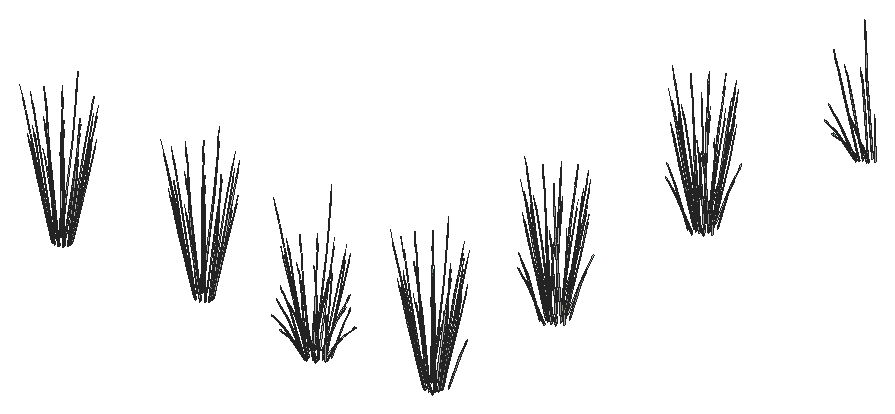
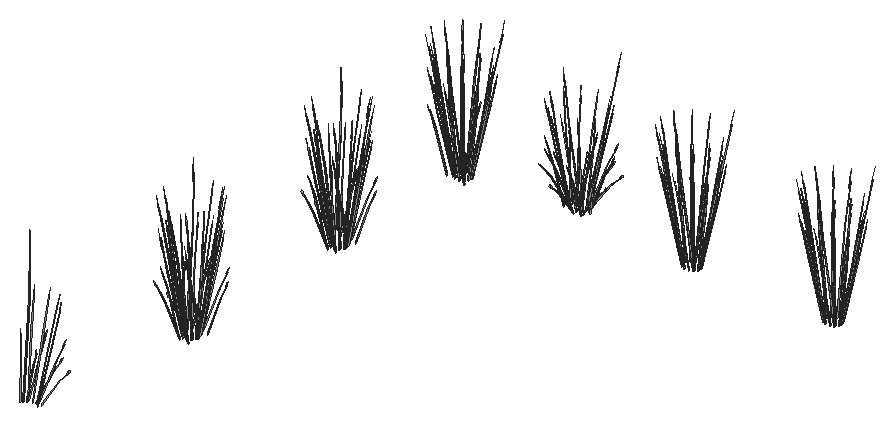
# SketchUp Ruby script. Lengths in inches.
U = 1.inch
M = Sketchup.active_model
def pt(a) = Geom::Point3d.new(a.map { |v| v * U })
def face(e, loops, mat)
  f = e.add_face(loops[0].map { |a| pt(a) })
  loops[1..].each { |l| e.add_face(l.map { |a| pt(a) }).erase! }
  f.material = f.back_material = mat if mat
  f
end
# faces: each face lists its corners as indices into pts; further lists are holes
def faces(e, pts, list, mat = nil) = list.each { |f| face(e, (f[0].is_a?(Array) ? f : [f]).map { |l| l.map { |i| pts[i] } }, mat) }
# xy, xz, yz: faces in a plane at the given z, y or x. An outline is a flat list of corners, or four numbers for a rectangle; further outlines are holes
def ring(l) = l.size == 4 ? [[l[0], l[1]], [l[2], l[1]], [l[2], l[3]], [l[0], l[3]]] : l.each_slice(2).to_a
def flat(e, list, mat, &to3) = list.each { |f| face(e, (f[0].is_a?(Array) ? f : [f]).map { |l| ring(l).map { |u, v| to3.(u, v) } }, mat) }
def xy(e, z, list, mat = nil) = flat(e, list, mat) { |x, y| [x, y, z] }
def xz(e, y, list, mat = nil) = flat(e, list, mat) { |x, z| [x, y, z] }
def yz(e, x, list, mat = nil) = flat(e, list, mat) { |y, z| [x, y, z] }
def lines(e, pts, list) = list.each { |a, b| e.add_line(pt(pts[a]), pt(pts[b])) }
# prism: a flat outline (further loops are holes) pulled along v
def prism(e, loops, v, mat = nil)
  f = face(e, loops, mat); d = Geom::Vector3d.new(v.map { |x| x * U })
  f.pushpull(f.normal.samedirection?(d) ? d.length : -d.length)
end
def box(e, o, s, mat = nil) = prism(e, [[o, [o[0] + s[0], o[1], o[2]], [o[0] + s[0], o[1] + s[1], o[2]], [o[0], o[1] + s[1], o[2]]]], [0, 0, s[2]], mat)
def at(x, y, z, deg = 0) = Geom::Transformation.translation(pt([x, y, z])) * Geom::Transformation.rotation(ORIGIN, Z_AXIS, deg.degrees)
def axes(o, x, y, z) = Geom::Transformation.new([*x, 0, *y, 0, *z, 0, *pt(o).to_a, 1])
def part(name) = M.definitions.add(name)
# library, detail: a bought-in or finely detailed component or shape, given as its bounding box
def library(name, o, s) = part(name).tap { |d| box(d.entities, o, s) }
def detail(e, o, s) = box(e.add_group.entities, o, s)
def put(e, d, t, mat = nil) = e.add_instance(d, t).tap { |i| i.material = mat if mat }
def group(e, t, mat = nil) = e.add_group.tap { |g| g.transformation = t; g.material = mat if mat }.entities
root = M.entities
M.materials.add("LightPink_Translucent").color = [175, 214, 192]
M.materials["LightPink_Translucent"].alpha = 0.75
c1 = part("blade")
p = [[2.15,0.21,22],[0,0.17,0],[0.09,0.45,0],[2.18,0.31,22],[2.29,0.31,22],[0.38,0.45,0],
  [2.48,0.24,33],[2.49,0.24,33],[2.48,0.22,33]]
faces(c1.entities,p,[[0,1,2,3],[4,5,2,3],[6,3,4,7],[8,0,3,6]])
c2 = part("seeds")
p = [[0.3,-0.1,1.38],[-0.01,-0.03,1.59],[-0.01,-0.03,0.03],[0.14,-0.07,-0.07],[0.29,-0.03,3],[0.15,0.01,3.11]]
faces(c2.entities,p,[[0,1,2,3],[1,0,4,5]],"LightPink_Translucent")
c3 = part("blade with seeds")
put(c3.entities,c1,at(0,0,0))
put(c3.entities,c2,axes([2.4,0.25,30.99],[1.5799,-0.05474,1.17369],[-0.12525,1.92788,0.29478],[-0.07173,-0.02425,1.56792]))
put(root,c3,axes([463.08,228.78,141.56],[-0.0731,-0.06244,1.59199],[-0.48785,0.03959,-0.25177],[-0.07786,-0.14934,0.12768]))
put(root,c3,axes([465.27,229.54,141.56],[-0.00461,-0.08863,1.59199],[-0.38966,-0.25616,-0.25177],[0.06024,-0.15528,0.12768]))
put(root,c3,axes([465.17,229.22,141.55],[-0.04854,0.03402,1.61419],[-0.47555,-0.11476,-0.15253],[-0.01722,-0.14844,0.28566]))
put(root,c3,axes([462.58,228.57,141.55],[-0.00892,0.05338,1.61419],[-0.43976,0.19372,-0.15253],[-0.12941,-0.09903,0.28566]))
put(root,c3,axes([463.81,229.57,141.57],[0.35217,-0.15135,0.05852],[0.17238,0.27599,0.46065],[-0.03401,-0.12166,0.70242]))
put(root,c3,axes([462.6,229.61,141.57],[0.21722,-0.2829,0.05852],[0.30933,0.1647,0.46065],[-0.10001,-0.0907,0.70242]))
put(root,c3,axes([462.7,229.59,142.21],[-0.31898,0.42693,-0.12394],[-0.46194,-0.24596,-0.6879],[-0.16057,-0.12062,1.04526]))
put(root,c3,axes([464.88,230.06,141.57],[0.39276,0.02075,0.05852],[-0.01077,0.31333,0.46065],[0.0411,-0.12002,0.70242]))
put(root,c3,axes([461.48,229.46,141.56],[-0.10283,-0.00314,1.59199],[-0.32739,0.31434,-0.25177],[-0.17468,-0.06423,0.12768]))
put(root,c3,axes([466.45,230.92,141.55],[-0.06243,-0.00338,1.61419],[-0.25923,-0.3624,-0.15253],[0.1041,-0.11916,0.28566]))
put(root,c3,axes([461.58,230.17,141.57],[0.02407,-0.33864,0.05852],[0.3634,0.00928,0.46065],[-0.13921,-0.03543,0.70242]))
put(root,c3,axes([465.52,230.9375,141.57],[0.32811,0.18729,0.05852],[-0.19103,0.26671,0.46065],[0.10519,-0.08623,0.70242]))
put(root,c3,axes([466.6875,231.35,141.56],[0.06632,-0.06783,1.59199],[-0.08489,-0.4161,-0.25177],[0.16641,-0.07889,0.12768]))
put(root,c3,axes([461.08,229.73,141.55],[0.03543,0.04444,1.61419],[-0.17081,0.3995,-0.15253],[-0.17299,0.00289,0.28566]))
put(root,c3,axes([461.02,231.09,141.57],[-0.17554,-0.30365,0.05852],[0.3201,-0.14862,0.46065],[-0.1411,0.02932,0.70242]))
put(root,c3,axes([492.89,234.04,141.46],[-0.04854,0.03402,1.61419],[-0.47555,-0.11476,-0.15253],[-0.01722,-0.14844,0.28566]))
put(root,c3,axes([465.57,231.98,141.57],[0.17554,0.30365,0.05852],[-0.3201,0.14862,0.46065],[0.1411,-0.02932,0.70242]))
put(root,c3,axes([391.2,234.42,141.48],[0.47094,0.11642,0.43682],[-0.16104,0.38276,0.36018],[-0.0283,-0.15052,0.9039]))
put(root,c3,axes([429.4,234.42,141.48],[0.47094,0.11642,0.43682],[-0.16104,0.38276,0.36018],[-0.0283,-0.15052,0.9039]))
put(root,c3,axes([491.41,234.42,141.48],[0.47094,0.11642,0.43682],[-0.16104,0.38276,0.36018],[-0.0283,-0.15052,0.9039]))
put(root,c3,axes([391.33,234.39,141.47],[0.35217,-0.15135,0.05852],[0.17238,0.27599,0.46065],[-0.03401,-0.12166,0.70242]))
put(root,c3,axes([429.52,234.39,141.47],[0.35217,-0.15135,0.05852],[0.17238,0.27599,0.46065],[-0.03401,-0.12166,0.70242]))
put(root,c3,axes([491.53,234.39,141.47],[0.35217,-0.15135,0.05852],[0.17238,0.27599,0.46065],[-0.03401,-0.12166,0.70242]))
put(root,c3,axes([390.12,234.43,141.47],[0.21722,-0.2829,0.05852],[0.30933,0.1647,0.46065],[-0.10001,-0.0907,0.70242]))
put(root,c3,axes([428.32,234.43,141.47],[0.21722,-0.2829,0.05852],[0.30933,0.1647,0.46065],[-0.10001,-0.0907,0.70242]))
put(root,c3,axes([490.33,234.43,141.47],[0.21722,-0.2829,0.05852],[0.30933,0.1647,0.46065],[-0.10001,-0.0907,0.70242]))
put(root,c3,axes([466.34,233.18,141.55],[-0.04322,-0.03899,1.61419],[0.09454,-0.41791,-0.15253],[0.17023,-0.0267,0.28566]))
put(root,c3,axes([460.71,231.49,141.56],[-0.07805,0.05782,1.59199],[0.00664,0.42244,-0.25177],[-0.1789,0.05494,0.12768]))
put(root,c3,axes([392.27,234.84,141.48],[0.34034,0.30385,0.43682],[-0.36143,0.26205,0.36018],[0.06278,-0.14256,0.9039]))
put(root,c3,axes([430.47,234.84,141.48],[0.34034,0.30385,0.43682],[-0.36143,0.26205,0.36018],[0.06278,-0.14256,0.9039]))
put(root,c3,axes([492.48,234.84,141.48],[0.34034,0.30385,0.43682],[-0.36143,0.26205,0.36018],[0.06278,-0.14256,0.9039]))
put(root,c3,axes([390.22,234.4,142.11],[-0.31898,0.42693,-0.12394],[-0.46194,-0.24596,-0.6879],[-0.16057,-0.12062,1.04526]))
put(root,c3,axes([428.41,234.4,142.11],[-0.31898,0.42693,-0.12394],[-0.46194,-0.24596,-0.6879],[-0.16057,-0.12062,1.04526]))
put(root,c3,axes([490.42,234.4,142.11],[-0.31898,0.42693,-0.12394],[-0.46194,-0.24596,-0.6879],[-0.16057,-0.12062,1.04526]))
put(root,c3,axes([392.4,234.875,141.47],[0.39276,0.02075,0.05852],[-0.01077,0.31333,0.46065],[0.0411,-0.12002,0.70242]))
put(root,c3,axes([430.59,234.875,141.47],[0.39276,0.02075,0.05852],[-0.01077,0.31333,0.46065],[0.0411,-0.12002,0.70242]))
put(root,c3,axes([492.6,234.875,141.47],[0.39276,0.02075,0.05852],[-0.01077,0.31333,0.46065],[0.0411,-0.12002,0.70242]))
put(root,c3,axes([465.26,232.55,141.56],[0.10253,-0.00753,1.59199],[0.28122,-0.34598,-0.25177],[0.18237,0.04567,0.12768]))
put(root,c3,axes([461.07,232.13,141.57],[-0.32811,-0.18729,0.05852],[0.19103,-0.26671,0.46065],[-0.10519,0.08623,0.70242]))
put(root,c3,axes([389.1,234.99,141.47],[0.02407,-0.33864,0.05852],[0.3634,0.00928,0.46065],[-0.13921,-0.03543,0.70242]))
put(root,c3,axes([427.3,234.99,141.47],[0.02407,-0.33864,0.05852],[0.3634,0.00928,0.46065],[-0.13921,-0.03543,0.70242]))
put(root,c3,axes([489.31,234.99,141.47],[0.02407,-0.33864,0.05852],[0.3634,0.00928,0.46065],[-0.13921,-0.03543,0.70242]))
put(root,c3,axes([459.85,231.91,141.55],[0.061,0.01194,1.61419],[0.18869,0.39348,-0.15253],[-0.12486,0.10328,0.28566]))
put(root,c3,axes([465.01,232.9,141.57],[-0.02407,0.33864,0.05852],[-0.3634,-0.00928,0.46065],[0.13921,0.03543,0.70242]))
put(root,c3,axes([393.04,235.75,141.47],[0.32811,0.18729,0.05852],[-0.19103,0.26671,0.46065],[0.10519,-0.08623,0.70242]))
put(root,c3,axes([431.24,235.75,141.47],[0.32811,0.18729,0.05852],[-0.19103,0.26671,0.46065],[0.10519,-0.08623,0.70242]))
put(root,c3,axes([493.25,235.75,141.47],[0.32811,0.18729,0.05852],[-0.19103,0.26671,0.46065],[0.10519,-0.08623,0.70242]))
put(root,c3,axes([392.95,235.67,141.48],[0.11853,0.40986,0.43682],[-0.46497,0.07113,0.36018],[0.13704,-0.09639,0.9039]))
put(root,c3,axes([431.15,235.67,141.48],[0.11853,0.40986,0.43682],[-0.46497,0.07113,0.36018],[0.13704,-0.09639,0.9039]))
put(root,c3,axes([493.16,235.67,141.48],[0.11853,0.40986,0.43682],[-0.46497,0.07113,0.36018],[0.13704,-0.09639,0.9039]))
put(root,c3,axes([463.51,233.63,141.55],[0.00141,-0.05392,1.61419],[0.40958,-0.23787,-0.15253],[0.14227,0.0849,0.28566]))
put(root,c3,axes([461.72,233.01,141.57],[-0.39276,-0.02075,0.05852],[0.01077,-0.31333,0.46065],[-0.0411,0.12002,0.70242]))
put(root,c3,axes([463.99,233.45,141.57],[-0.21722,0.2829,0.05852],[-0.30933,-0.1647,0.46065],[0.10001,0.0907,0.70242]))
put(root,c3,axes([462.79,233.5,141.57],[-0.35217,0.15135,0.05852],[-0.17238,-0.27599,0.46065],[0.03401,0.12166,0.70242]))
put(root,c3,axes([460.73,233.0625,141.56],[-0.01188,0.08813,1.59199],[0.33715,0.30658,-0.25177],[-0.08826,0.14498,0.12768]))
put(root,c3,axes([461.8,232.87,142.18],[0.52527,0.02206,-0.12283],[-0.01436,0.41777,-0.68176],[-0.03649,0.1609,1.03593]))
put(root,c3,axes([388.57,236.02,141.48],[0.13503,-0.40605,0.43682],[0.44393,0.13885,0.36018],[-0.17458,0.0244,0.9039]))
put(root,c3,axes([426.77,236.02,141.48],[0.13503,-0.40605,0.43682],[0.44393,0.13885,0.36018],[-0.17458,0.0244,0.9039]))
put(root,c3,axes([488.78,236.02,141.48],[0.13503,-0.40605,0.43682],[0.44393,0.13885,0.36018],[-0.17458,0.0244,0.9039]))
put(root,c3,axes([388.54,235.91,141.47],[-0.17554,-0.30365,0.05852],[0.3201,-0.14862,0.46065],[-0.1411,0.02932,0.70242]))
put(root,c3,axes([426.73,235.91,141.47],[-0.17554,-0.30365,0.05852],[0.3201,-0.14862,0.46065],[-0.1411,0.02932,0.70242]))
put(root,c3,axes([488.75,235.91,141.47],[-0.17554,-0.30365,0.05852],[0.3201,-0.14862,0.46065],[-0.1411,0.02932,0.70242]))
put(root,c3,axes([460.6875,233.97,141.55],[0.05422,-0.02689,1.61419],[0.44816,0.17884,-0.15253],[-0.01053,0.14891,0.28566]))
put(root,c3,axes([393.09,236.79,141.47],[0.17554,0.30365,0.05852],[-0.3201,0.14862,0.46065],[0.1411,-0.02932,0.70242]))
put(root,c3,axes([431.29,236.79,141.47],[0.17554,0.30365,0.05852],[-0.3201,0.14862,0.46065],[0.1411,-0.02932,0.70242]))
put(root,c3,axes([493.3,236.79,141.47],[0.17554,0.30365,0.05852],[-0.3201,0.14862,0.46065],[0.1411,-0.02932,0.70242]))
put(root,c3,axes([393.06,236.6875,141.48],[-0.13503,0.40605,0.43682],[-0.44393,-0.13885,0.36018],[0.17458,-0.0244,0.9039]))
put(root,c3,axes([431.25,236.6875,141.48],[-0.13503,0.40605,0.43682],[-0.44393,-0.13885,0.36018],[0.17458,-0.0244,0.9039]))
put(root,c3,axes([493.26,236.6875,141.48],[-0.13503,0.40605,0.43682],[-0.44393,-0.13885,0.36018],[0.17458,-0.0244,0.9039]))
put(root,c3,axes([462.67,234.15,141.56],[0.06058,0.07171,1.59199],[0.48891,0.02817,-0.25177],[0.04916,0.15815,0.12768]))
put(root,c3,axes([494.0625,238,141.46],[-0.04322,-0.03899,1.61419],[0.09454,-0.41791,-0.15253],[0.17023,-0.0267,0.28566]))
put(root,c3,axes([388.68,237.03,141.48],[-0.11853,-0.40986,0.43682],[0.46497,-0.07113,0.36018],[-0.13704,0.09639,0.9039]))
put(root,c3,axes([426.875,237.03,141.48],[-0.11853,-0.40986,0.43682],[0.46497,-0.07113,0.36018],[-0.13704,0.09639,0.9039]))
put(root,c3,axes([488.89,237.03,141.48],[-0.11853,-0.40986,0.43682],[0.46497,-0.07113,0.36018],[-0.13704,0.09639,0.9039]))
put(root,c3,axes([388.59,236.95,141.47],[-0.32811,-0.18729,0.05852],[0.19103,-0.26671,0.46065],[-0.10519,0.08623,0.70242]))
put(root,c3,axes([426.78,236.95,141.47],[-0.32811,-0.18729,0.05852],[0.19103,-0.26671,0.46065],[-0.10519,0.08623,0.70242]))
put(root,c3,axes([488.79,236.95,141.47],[-0.32811,-0.18729,0.05852],[0.19103,-0.26671,0.46065],[-0.10519,0.08623,0.70242]))
put(root,c3,axes([392.53,237.72,141.47],[-0.02407,0.33864,0.05852],[-0.3634,-0.00928,0.46065],[0.13921,0.03543,0.70242]))
put(root,c3,axes([430.73,237.72,141.47],[-0.02407,0.33864,0.05852],[-0.3634,-0.00928,0.46065],[0.13921,0.03543,0.70242]))
put(root,c3,axes([492.74,237.72,141.47],[-0.02407,0.33864,0.05852],[-0.3634,-0.00928,0.46065],[0.13921,0.03543,0.70242]))
put(root,c3,axes([392.5625,237.61,141.48],[-0.35241,0.29344,0.43682],[-0.30393,-0.31162,0.36018],[0.16534,0.05413,0.9039]))
put(root,c3,axes([430.76,237.61,141.48],[-0.35241,0.29344,0.43682],[-0.30393,-0.31162,0.36018],[0.16534,0.05413,0.9039]))
put(root,c3,axes([492.77,237.61,141.48],[-0.35241,0.29344,0.43682],[-0.30393,-0.31162,0.36018],[0.16534,0.05413,0.9039]))
put(root,c3,axes([389.23,237.83,141.47],[-0.39276,-0.02075,0.05852],[0.01077,-0.31333,0.46065],[-0.0411,0.12002,0.70242]))
put(root,c3,axes([427.43,237.83,141.47],[-0.39276,-0.02075,0.05852],[0.01077,-0.31333,0.46065],[-0.0411,0.12002,0.70242]))
put(root,c3,axes([489.44,237.83,141.47],[-0.39276,-0.02075,0.05852],[0.01077,-0.31333,0.46065],[-0.0411,0.12002,0.70242]))
put(root,c3,axes([389.36,237.86,141.48],[-0.34034,-0.30385,0.43682],[0.36143,-0.26205,0.36018],[-0.06278,0.14256,0.9039]))
put(root,c3,axes([427.55,237.86,141.48],[-0.34034,-0.30385,0.43682],[0.36143,-0.26205,0.36018],[-0.06278,0.14256,0.9039]))
put(root,c3,axes([489.57,237.86,141.48],[-0.34034,-0.30385,0.43682],[0.36143,-0.26205,0.36018],[-0.06278,0.14256,0.9039]))
put(root,c3,axes([391.51,238.27,141.47],[-0.21722,0.2829,0.05852],[-0.30933,-0.1647,0.46065],[0.10001,0.0907,0.70242]))
put(root,c3,axes([429.71,238.27,141.47],[-0.21722,0.2829,0.05852],[-0.30933,-0.1647,0.46065],[0.10001,0.0907,0.70242]))
put(root,c3,axes([491.72,238.27,141.47],[-0.21722,0.2829,0.05852],[-0.30933,-0.1647,0.46065],[0.10001,0.0907,0.70242]))
put(root,c3,axes([391.6,238.19,141.48],[-0.47536,0.1022,0.43682],[-0.0825,-0.4009,0.36018],[0.1118,0.11815,0.9039]))
put(root,c3,axes([429.8,238.19,141.48],[-0.47536,0.1022,0.43682],[-0.0825,-0.4009,0.36018],[0.1118,0.11815,0.9039]))
put(root,c3,axes([491.81,238.19,141.48],[-0.47536,0.1022,0.43682],[-0.0825,-0.4009,0.36018],[0.1118,0.11815,0.9039]))
put(root,c3,axes([390.3,238.31,141.47],[-0.35217,0.15135,0.05852],[-0.17238,-0.27599,0.46065],[0.03401,0.12166,0.70242]))
put(root,c3,axes([428.5,238.31,141.47],[-0.35217,0.15135,0.05852],[-0.17238,-0.27599,0.46065],[0.03401,0.12166,0.70242]))
put(root,c3,axes([490.51,238.31,141.47],[-0.35217,0.15135,0.05852],[-0.17238,-0.27599,0.46065],[0.03401,0.12166,0.70242]))
put(root,c3,axes([389.32,237.68,142.08],[0.52527,0.02206,-0.12283],[-0.01436,0.41777,-0.68176],[-0.03649,0.1609,1.03593]))
put(root,c3,axes([427.52,237.68,142.08],[0.52527,0.02206,-0.12283],[-0.01436,0.41777,-0.68176],[-0.03649,0.1609,1.03593]))
put(root,c3,axes([489.53,237.68,142.08],[0.52527,0.02206,-0.12283],[-0.01436,0.41777,-0.68176],[-0.03649,0.1609,1.03593]))
put(root,c3,axes([488.41,238.79,141.46],[0.05422,-0.02689,1.61419],[0.44816,0.17884,-0.15253],[-0.01053,0.14891,0.28566]))
put(root,c3,axes([492.64,272.05,141.46],[-0.01194,0.061,1.61419],[-0.39348,0.18869,-0.15253],[-0.10328,-0.12486,0.28566]))
put(root,c3,axes([494.83,273.29,141.46],[-0.04444,0.03543,1.61419],[-0.3995,-0.17081,-0.15253],[-0.00289,-0.17299,0.28566]))
put(root,c3,axes([493.36,273.26,141.48],[0.40605,0.13503,0.43682],[-0.13885,0.44393,0.36018],[-0.0244,-0.17458,0.9039]))
put(root,c3,axes([493.46,273.22,141.47],[0.30365,-0.17554,0.05852],[0.14862,0.3201,0.46065],[-0.02932,-0.1411,0.70242]))
put(root,c3,axes([492.35,273.37,141.48],[0.40986,-0.11853,0.43682],[0.07113,0.46497,0.36018],[-0.09639,-0.13704,0.9039]))
put(root,c3,axes([492.42,273.27,141.47],[0.18729,-0.32811,0.05852],[0.26671,0.19103,0.46065],[-0.08623,-0.10519,0.70242]))
put(root,c3,axes([494.39,273.79,141.47],[0.33864,0.02407,0.05852],[-0.00928,0.3634,0.46065],[0.03543,-0.13921,0.70242]))
put(root,c3,axes([494.97,274.9,142.11],[-0.42693,-0.31898,-0.12394],[0.24596,-0.46194,-0.6879],[0.12062,-0.16057,1.04526]))
put(root,c3,axes([495.99,274.78,141.46],[-0.05338,-0.00892,1.61419],[-0.19372,-0.43976,-0.15253],[0.09903,-0.12941,0.28566]))
put(root,c3,axes([491.52,274.04,141.48],[0.30385,-0.34034,0.43682],[0.26205,0.36143,0.36018],[-0.14256,-0.06278,0.9039]))
put(root,c3,axes([491.54,273.92,141.47],[0.02075,-0.39276,0.05852],[0.31333,0.01077,0.46065],[-0.12002,-0.0411,0.70242]))
put(root,c3,axes([490.59,272.89,141.46],[0.02689,0.05422,1.61419],[-0.17884,0.44816,-0.15253],[-0.14891,-0.01053,0.28566]))
put(root,c3,axes([494.94,274.81,141.47],[0.2829,0.21722,0.05852],[-0.1647,0.30933,0.46065],[0.0907,-0.10001,0.70242]))
put(root,c3,axes([491.69,274.01,142.08],[-0.02206,0.52527,-0.12283],[-0.41777,-0.01436,-0.68176],[-0.1609,-0.03649,1.03593]))
put(root,c3,axes([491.0625,274.99,141.47],[-0.15135,-0.35217,0.05852],[0.27599,-0.17238,0.46065],[-0.12166,0.03401,0.70242]))
put(root,c3,axes([494.99,276.01,141.47],[0.15135,0.35217,0.05852],[-0.27599,0.17238,0.46065],[0.12166,-0.03401,0.70242]))
put(root,c3,axes([494.96,275.89,141.48],[-0.11642,0.47094,0.43682],[-0.38276,-0.16104,0.36018],[0.15052,-0.0283,0.9039]))
put(root,c3,axes([495.34,277.37,141.46],[-0.03402,-0.04854,1.61419],[0.11476,-0.47555,-0.15253],[0.14844,-0.01722,0.28566]))
put(root,c3,axes([491.18,276.29,141.48],[-0.1022,-0.47536,0.43682],[0.4009,-0.0825,0.36018],[-0.11815,0.1118,0.9039]))
put(root,c3,axes([491.1,276.2,141.47],[-0.2829,-0.21722,0.05852],[0.1647,-0.30933,0.46065],[-0.0907,0.10001,0.70242]))
put(root,c3,axes([490.93,275.72,141.46],[0.05392,0.00141,1.61419],[0.23787,0.40958,-0.15253],[-0.0849,0.14227,0.28566]))
put(root,c3,axes([494.5,277.08,141.47],[-0.02075,0.39276,0.05852],[-0.31333,-0.01077,0.46065],[0.12002,0.0411,0.70242]))
put(root,c3,axes([494.53,276.96,141.48],[-0.30385,0.34034,0.43682],[-0.26205,-0.36143,0.36018],[0.14256,0.06278,0.9039]))
put(root,c3,axes([491.66,277.22,141.47],[-0.33864,-0.02407,0.05852],[0.00928,-0.3634,0.46065],[-0.03543,0.13921,0.70242]))
put(root,c3,axes([491.77,277.25,141.48],[-0.29344,-0.35241,0.43682],[0.31162,-0.30393,0.36018],[-0.05413,0.16534,0.9039]))
put(root,c3,axes([493.62,277.73,141.47],[-0.18729,0.32811,0.05852],[-0.26671,-0.19103,0.46065],[0.08623,0.10519,0.70242]))
put(root,c3,axes([493.7,277.64,141.48],[-0.40986,0.11853,0.43682],[-0.07113,-0.46497,0.36018],[0.09639,0.13704,0.9039]))
put(root,c3,axes([493.64,278.65,141.46],[0.00338,-0.06243,1.61419],[0.3624,-0.25923,-0.15253],[0.11916,0.1041,0.28566]))
put(root,c3,axes([492.58,277.78,141.47],[-0.30365,0.17554,0.05852],[-0.14862,-0.3201,0.46065],[0.02932,0.1411,0.70242]))
put(root,c3,axes([492.6875,277.74,141.48],[-0.40605,-0.13503,0.43682],[0.13885,-0.44393,0.36018],[0.0244,0.17458,0.9039]))
put(root,c3,axes([491.375,278.54,141.46],[0.03899,-0.04322,1.61419],[0.41791,0.09454,-0.15253],[0.0267,0.17023,0.28566]))
put(root,c3,axes([492.64,322.04,141.46],[-0.01194,0.061,1.61419],[-0.39348,0.18869,-0.15253],[-0.10328,-0.12486,0.28566]))
put(root,c3,axes([494.83,323.27,141.46],[-0.04444,0.03543,1.61419],[-0.3995,-0.17081,-0.15253],[-0.00289,-0.17299,0.28566]))
put(root,c3,axes([493.36,323.25,141.48],[0.40605,0.13503,0.43682],[-0.13885,0.44393,0.36018],[-0.0244,-0.17458,0.9039]))
put(root,c3,axes([493.46,323.21,141.47],[0.30365,-0.17554,0.05852],[0.14862,0.3201,0.46065],[-0.02932,-0.1411,0.70242]))
put(root,c3,axes([492.35,323.35,141.48],[0.40986,-0.11853,0.43682],[0.07113,0.46497,0.36018],[-0.09639,-0.13704,0.9039]))
put(root,c3,axes([492.42,323.26,141.47],[0.18729,-0.32811,0.05852],[0.26671,0.19103,0.46065],[-0.08623,-0.10519,0.70242]))
put(root,c3,axes([494.39,323.77,141.47],[0.33864,0.02407,0.05852],[-0.00928,0.3634,0.46065],[0.03543,-0.13921,0.70242]))
put(root,c3,axes([494.97,324.89,142.11],[-0.42693,-0.31898,-0.12394],[0.24596,-0.46194,-0.6879],[0.12062,-0.16057,1.04526]))
put(root,c3,axes([495.99,324.77,141.46],[-0.05338,-0.00892,1.61419],[-0.19372,-0.43976,-0.15253],[0.09903,-0.12941,0.28566]))
put(root,c3,axes([491.52,324.03,141.48],[0.30385,-0.34034,0.43682],[0.26205,0.36143,0.36018],[-0.14256,-0.06278,0.9039]))
put(root,c3,axes([491.54,323.91,141.47],[0.02075,-0.39276,0.05852],[0.31333,0.01077,0.46065],[-0.12002,-0.0411,0.70242]))
put(root,c3,axes([490.59,322.88,141.46],[0.02689,0.05422,1.61419],[-0.17884,0.44816,-0.15253],[-0.14891,-0.01053,0.28566]))
put(root,c3,axes([494.94,324.79,141.47],[0.2829,0.21722,0.05852],[-0.1647,0.30933,0.46065],[0.0907,-0.10001,0.70242]))
put(root,c3,axes([491.69,323.99,142.08],[-0.02206,0.52527,-0.12283],[-0.41777,-0.01436,-0.68176],[-0.1609,-0.03649,1.03593]))
put(root,c3,axes([491.0625,324.98,141.47],[-0.15135,-0.35217,0.05852],[0.27599,-0.17238,0.46065],[-0.12166,0.03401,0.70242]))
put(root,c3,axes([494.99,326,141.47],[0.15135,0.35217,0.05852],[-0.27599,0.17238,0.46065],[0.12166,-0.03401,0.70242]))
put(root,c3,axes([494.96,325.875,141.48],[-0.11642,0.47094,0.43682],[-0.38276,-0.16104,0.36018],[0.15052,-0.0283,0.9039]))
put(root,c3,axes([495.34,327.36,141.46],[-0.03402,-0.04854,1.61419],[0.11476,-0.47555,-0.15253],[0.14844,-0.01722,0.28566]))
put(root,c3,axes([491.18,326.27,141.48],[-0.1022,-0.47536,0.43682],[0.4009,-0.0825,0.36018],[-0.11815,0.1118,0.9039]))
put(root,c3,axes([491.1,326.18,141.47],[-0.2829,-0.21722,0.05852],[0.1647,-0.30933,0.46065],[-0.0907,0.10001,0.70242]))
put(root,c3,axes([490.93,325.71,141.46],[0.05392,0.00141,1.61419],[0.23787,0.40958,-0.15253],[-0.0849,0.14227,0.28566]))
put(root,c3,axes([494.5,327.07,141.47],[-0.02075,0.39276,0.05852],[-0.31333,-0.01077,0.46065],[0.12002,0.0411,0.70242]))
put(root,c3,axes([494.53,326.94,141.48],[-0.30385,0.34034,0.43682],[-0.26205,-0.36143,0.36018],[0.14256,0.06278,0.9039]))
put(root,c3,axes([491.66,327.2,141.47],[-0.33864,-0.02407,0.05852],[0.00928,-0.3634,0.46065],[-0.03543,0.13921,0.70242]))
put(root,c3,axes([491.77,327.24,141.48],[-0.29344,-0.35241,0.43682],[0.31162,-0.30393,0.36018],[-0.05413,0.16534,0.9039]))
put(root,c3,axes([493.62,327.72,141.47],[-0.18729,0.32811,0.05852],[-0.26671,-0.19103,0.46065],[0.08623,0.10519,0.70242]))
put(root,c3,axes([493.7,327.625,141.48],[-0.40986,0.11853,0.43682],[-0.07113,-0.46497,0.36018],[0.09639,0.13704,0.9039]))
put(root,c3,axes([493.64,328.64,141.46],[0.00338,-0.06243,1.61419],[0.3624,-0.25923,-0.15253],[0.11916,0.1041,0.28566]))
put(root,c3,axes([492.58,327.76,141.47],[-0.30365,0.17554,0.05852],[-0.14862,-0.3201,0.46065],[0.02932,0.1411,0.70242]))
put(root,c3,axes([492.6875,327.73,141.48],[-0.40605,-0.13503,0.43682],[0.13885,-0.44393,0.36018],[0.0244,0.17458,0.9039]))
put(root,c3,axes([491.375,328.53,141.46],[0.03899,-0.04322,1.61419],[0.41791,0.09454,-0.15253],[0.0267,0.17023,0.28566]))
put(root,c3,axes([500.51,368.81,141.56],[-0.05782,-0.07805,1.59199],[-0.42244,0.00664,-0.25177],[-0.05494,-0.1789,0.12768]))
put(root,c3,axes([500.09,367.94,141.55],[-0.01194,0.061,1.61419],[-0.39348,0.18869,-0.15253],[-0.10328,-0.12486,0.28566]))
put(root,c3,axes([502.27,369.18,141.55],[-0.04444,0.03543,1.61419],[-0.3995,-0.17081,-0.15253],[-0.00289,-0.17299,0.28566]))
put(root,c3,axes([502.54,369.58,141.56],[0.00314,-0.10283,1.59199],[-0.31434,-0.32739,-0.25177],[0.06423,-0.17468,0.12768]))
put(root,c3,axes([500.91,369.12,141.57],[0.30365,-0.17554,0.05852],[0.14862,0.3201,0.46065],[-0.02932,-0.1411,0.70242]))
put(root,c3,axes([499.87,369.17,141.57],[0.18729,-0.32811,0.05852],[0.26671,0.19103,0.46065],[-0.08623,-0.10519,0.70242]))
put(root,c3,axes([501.83,369.68,141.57],[0.33864,0.02407,0.05852],[-0.00928,0.3634,0.46065],[0.03543,-0.13921,0.70242]))
put(root,c3,axes([498.9375,368.82,141.56],[-0.08813,-0.01188,1.59199],[-0.30658,0.33715,-0.25177],[-0.14498,-0.08826,0.12768]))
put(root,c3,axes([502.41,370.8,142.21],[-0.42693,-0.31898,-0.12394],[0.24596,-0.46194,-0.6879],[0.12062,-0.16057,1.04526]))
put(root,c3,axes([503.43,370.67,141.55],[-0.05338,-0.00892,1.61419],[-0.19372,-0.43976,-0.15253],[0.09903,-0.12941,0.28566]))
put(root,c3,axes([498.99,369.8125,141.57],[0.02075,-0.39276,0.05852],[0.31333,0.01077,0.46065],[-0.12002,-0.0411,0.70242]))
